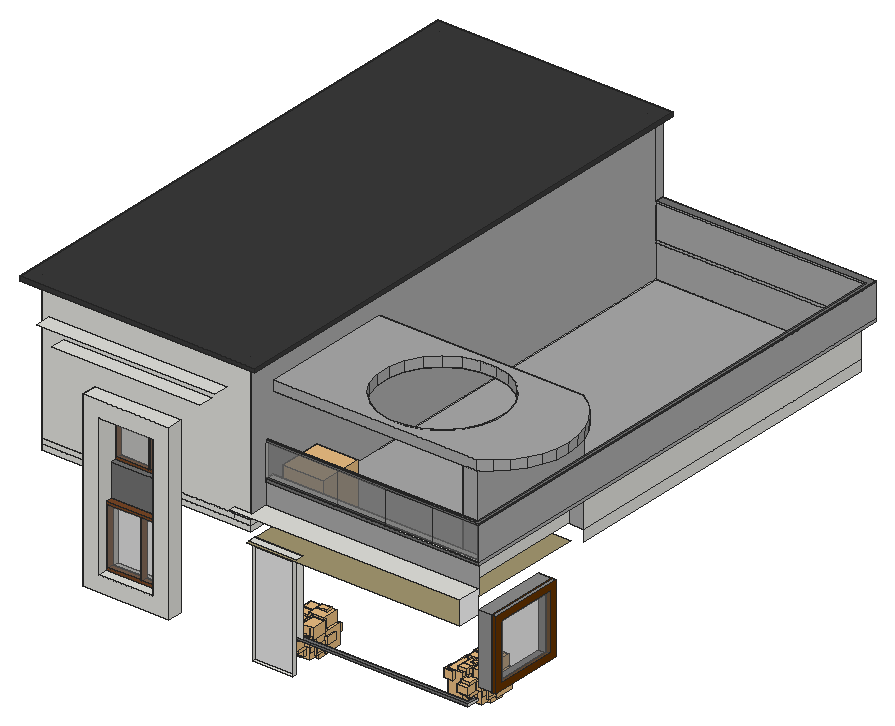
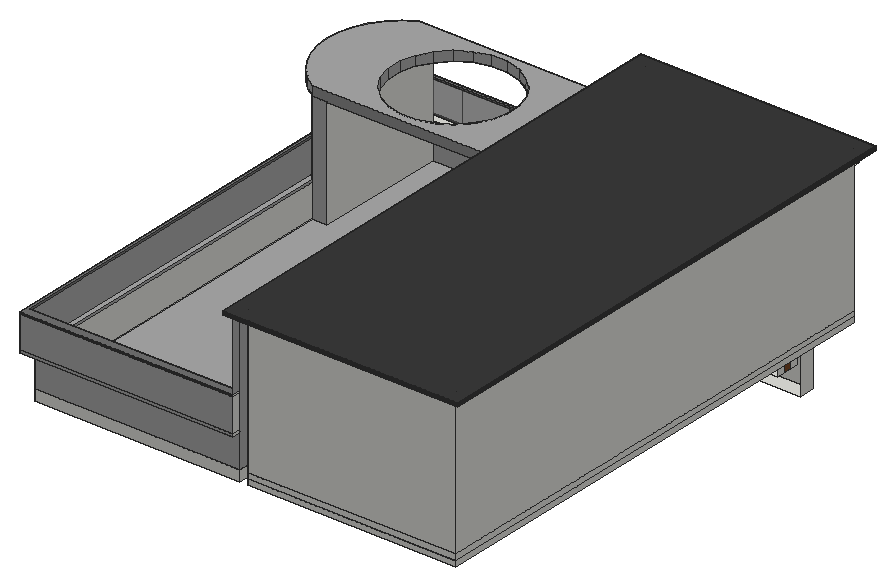
# SketchUp Ruby script. Lengths in inches.
U = 1.inch
M = Sketchup.active_model
def pt(a) = Geom::Point3d.new(a.map { |v| v * U })
def face(e, loops, mat)
  f = e.add_face(loops[0].map { |a| pt(a) })
  loops[1..].each { |l| e.add_face(l.map { |a| pt(a) }).erase! }
  f.material = f.back_material = mat if mat
  f
end
# faces: each face lists its corners as indices into pts; further lists are holes
def faces(e, pts, list, mat = nil) = list.each { |f| face(e, (f[0].is_a?(Array) ? f : [f]).map { |l| l.map { |i| pts[i] } }, mat) }
# xy, xz, yz: faces in a plane at the given z, y or x. An outline is a flat list of corners, or four numbers for a rectangle; further outlines are holes
def ring(l) = l.size == 4 ? [[l[0], l[1]], [l[2], l[1]], [l[2], l[3]], [l[0], l[3]]] : l.each_slice(2).to_a
def flat(e, list, mat, &to3) = list.each { |f| face(e, (f[0].is_a?(Array) ? f : [f]).map { |l| ring(l).map { |u, v| to3.(u, v) } }, mat) }
def xy(e, z, list, mat = nil) = flat(e, list, mat) { |x, y| [x, y, z] }
def xz(e, y, list, mat = nil) = flat(e, list, mat) { |x, z| [x, y, z] }
def yz(e, x, list, mat = nil) = flat(e, list, mat) { |y, z| [x, y, z] }
def lines(e, pts, list) = list.each { |a, b| e.add_line(pt(pts[a]), pt(pts[b])) }
# prism: a flat outline (further loops are holes) pulled along v
def prism(e, loops, v, mat = nil)
  f = face(e, loops, mat); d = Geom::Vector3d.new(v.map { |x| x * U })
  f.pushpull(f.normal.samedirection?(d) ? d.length : -d.length)
end
def box(e, o, s, mat = nil) = prism(e, [[o, [o[0] + s[0], o[1], o[2]], [o[0] + s[0], o[1] + s[1], o[2]], [o[0], o[1] + s[1], o[2]]]], [0, 0, s[2]], mat)
def at(x, y, z, deg = 0) = Geom::Transformation.translation(pt([x, y, z])) * Geom::Transformation.rotation(ORIGIN, Z_AXIS, deg.degrees)
def axes(o, x, y, z) = Geom::Transformation.new([*x, 0, *y, 0, *z, 0, *pt(o).to_a, 1])
def part(name) = M.definitions.add(name)
# library, detail: a bought-in or finely detailed component or shape, given as its bounding box
def library(name, o, s) = part(name).tap { |d| box(d.entities, o, s) }
def detail(e, o, s) = box(e.add_group.entities, o, s)
def put(e, d, t, mat = nil) = e.add_instance(d, t).tap { |i| i.material = mat if mat }
def group(e, t, mat = nil) = e.add_group.tap { |g| g.transformation = t; g.material = mat if mat }.entities
root = M.entities
M.materials.add("Bud_1").color = [142, 54, 77]
M.materials.add("Bud_2").color = [160, 82, 113]
M.materials.add("Bud_3").color = [186, 134, 155]
M.materials.add("Peony_Br1").color = [26, 30, 15]
M.materials.add("[Color C08]1").color = [102, 51, 0]
M.materials.add("[Color M00]").color = [255, 255, 255]
M.materials.add("[Color M03]").color = [170, 170, 170]
M.materials.add("[Color M04]").color = [142, 142, 142]
M.materials.add("[Color M05]").color = [114, 114, 114]
M.materials.add("[Color M07]").color = [58, 58, 58]
M.materials.add("[Sketchy Scales]").color = [229, 229, 229]
M.materials.add("[Translucent Glass Gray]").color = [128, 128, 128]
M.materials["[Translucent Glass Gray]"].alpha = 0.5
M.materials.add("[Wood Lumber ButtJoined]").color = [164, 152, 112]
M.materials.add("[Wood Veneer 01]").color = [120, 70, 37]
c1 = library("Group\#61",[-54.58,-83.54,30.99],[209.74,138.81,269.85])
c2 = library("Group\#54",[-161.17,-232.45,32.75],[152.53,236.06,399.97])
c3 = library("Group\#58",[-62.72,-147.62,57.55],[93.45,86.61,60.22])
c4 = library("Group\#55",[6.78,-176.96,61.53],[128.84,205.63,400.02])
c5 = library("Group\#60",[-32.97,-25.89,74.09],[206.79,187.79,274.23])
c6 = library("Group\#56",[-1.6875,-94.42,75.86],[134.92,113.41,305.11])
c7 = library("Group\#57",[-60.84,-159.99,77.97],[92.87,130.98,190.36])
c8 = library("Group\#59",[-84.97,-34.6875,78.05],[116.39,151.55,263.18])
c9 = library("Group\#14",[-14.51,-199.73,94.2],[105.22,97.74,77.03])
c10 = library("Group\#13",[-28.1,-125.85,106.48],[194.72,128.52,261.01])
c11 = library("Group\#15",[-24.89,-182.93,111.64],[113.72,173.94,173.74])
c12 = library("Group\#51",[-39.88,-92.9,113.08],[80.99,54.06,154.09])
c13 = library("Group\#36",[-37.32,-33.18,117.69],[148.47,104.95,286.6])
c14 = library("Group\#6",[-53.74,7.67,120.98],[106.95,236.74,251.98])
c15 = library("Group\#32",[-118.71,-26.72,138.49],[113,166.64,338.37])
c16 = library("Group\#30",[-110.02,-64.26,144.44],[128.07,118.55,275.77])
c17 = library("Group\#18",[-21.74,-164.88,146.75],[158.66,158.69,243.45])
c18 = library("Group\#9",[-100.48,19.53,147.87],[113.05,111.28,101.19])
c19 = library("Group\#12",[70.77,-125.64,148.84],[102.7,108.07,96.82])
c20 = library("Group\#34",[-136.13,-14.65,175.64],[147.69,202.17,192.49])
c21 = library("Group\#17",[2.57,-271.06,187.04],[93.4,209.89,191.26])
c22 = library("Group\#125",[134.07,-35.59,197.42],[66.93,108.39,101.45])
c23 = library("Group\#42",[-81.93,-128.91,211.16],[107.53,90.8,94.63])
c24 = library("Group\#28",[-168.05,-105.3,214.4],[173.05,109.74,165.51])
c25 = library("Group\#24",[-86.85,-171.15,214.86],[148.39,157.28,240.38])
c26 = library("Group\#124",[44.02,93.6,218.34],[115.22,101.76,105.18])
c27 = library("Group\#38",[-20.13,5.57,225.44],[155.68,162.88,267.12])
c28 = library("Group\#16",[-7.79,-309.02,238.22],[108.5,93.72,102.44])
c29 = library("Group\#126",[-107.16,-137.18,245.54],[76.51,112.05,84.97])
c30 = library("Group\#19",[51.13,-202.98,245.86],[103.83,96.91,120.11])
c31 = library("Group\#48",[1.16,-23.73,246.66],[101.27,126.17,86.62])
c32 = library("Group\#10",[-54.85,-171.1875,247.55],[90.72,132.3,71.07])
c33 = library("Group\#50",[-94.36,-157.31,255.2],[101.84,115.08,71.07])
c34 = library("Group\#31",[-124.14,3.49,256.66],[120.45,70.64,46.18])
c35 = library("Group\#33",[-159.97,129.63,257.39],[89.36,80.73,106.4])
c36 = library("Group\#39",[-80.73,-182.31,261.98],[90.74,132.73,71.97])
c37 = library("Group\#53",[-39.96,0.65,262.91],[71.32,151.8,74.06])
c38 = library("Group\#22",[-80.82,10.33,268.03],[91.87,74,84.35])
c39 = library("Group\#45",[-10.36,3.03,272.26],[79.07,139.88,53.94])
c40 = library("Group\#44",[-45.26,-82.43,273.6875],[73.19,105.45,181.93])
c41 = library("Group\#47",[-40.71,1.11,275.78],[91.4,147.63,75.64])
c42 = library("Group\#27",[-210.125,-102.4375,276.88],[51.54,90.91,87.28])
c43 = library("Group\#123",[-19.56,232.65,283.18],[66.82,42.19,66.65])
c44 = library("Group\#41",[-39.42,-209.09,286.91],[66.94,168.34,116.98])
c45 = library("Group\#8",[-56.625,3.66,294.95],[88.3,152.82,59.14])
c46 = library("Group\#49",[-53.8125,-212.33,295.34],[68.49,139.76,73.67])
c47 = library("Group\#46",[24.16,-5.45,296.62],[84.08,128.04,53.21])
c48 = library("Group\#25",[-191.98,-250.23,297.57],[97.9,89.36,114.5])
c49 = library("Group\#52",[-59.78,14.09,300.39],[101.06,171.37,85.05])
c50 = library("Group\#20",[111.16,-90.29,303.89],[49.95,90,76.18])
c51 = library("Group\#26",[-192.01,-26.24,304.89],[187.25,107.21,53.21])
c52 = library("Group\#40",[-75.53,-189.01,309.71],[68.94,147.24,88.69])
c53 = library("Group\#43",[-21.54,14.12,313.18],[84.79,137.02,109.55])
c54 = library("Group\#11",[-161.51,-101.97,314.73],[172.81,108.71,69.27])
c55 = library("Group\#7",[-49.75,139.84,314.95],[22.11,22.61,22.06])
c56 = library("Group\#21",[47.44,-177.11,343.1],[125.1,149.08,142.01])
c57 = library("Group\#29",[-147.09,-43.87,347.03],[63.89,87.81,80.15])
c58 = library("Group\#35",[-5.59,-15.12,374.79],[85.57,86.81,59.51])
c59 = library("Group\#127",[-126.0625,56.51,376.27],[112.05,106.35,108.99])
c60 = library("Group\#23",[-75.58,-212.0625,396.64],[87.14,69.73,75.82])
c61 = library("Group\#37",[-6.61,93.85,461.94],[98.68,62.42,49.38])
c62 = part("Group\#3")
xy(c62.entities,0,[[0,0,47.875,6]])
xy(c62.entities,1.8,[[1.8,0,30.57,6],[31.73,0,46.07,6]],"[Wood Veneer 01]")
xy(c62.entities,34.82,[[1.8,0,30.57,6],[31.73,0,46.07,6]])
xy(c62.entities,36.625,[[0,0,47.875,6]],"[Wood Veneer 01]")
xz(c62.entities,0,[[1.8,1.8,30.57,34.82],[31.73,1.8,46.07,34.82]],"[Translucent Glass Gray]")
xz(c62.entities,0,[[[0,0,47.875,36.625],[1.8,1.8,30.57,34.82],[31.73,1.8,46.07,34.82]]],"[Wood Veneer 01]")
xz(c62.entities,6,[[[0,0,47.875,36.625],[1.8,1.8,30.57,34.82],[31.73,1.8,46.07,34.82]]],"[Wood Veneer 01]")
yz(c62.entities,0,[[0,0,6,36.625]],"[Wood Veneer 01]")
yz(c62.entities,1.8,[[0,1.8,6,34.82]],"[Wood Veneer 01]")
yz(c62.entities,30.57,[[0,1.8,6,34.82]],"[Wood Veneer 01]")
yz(c62.entities,31.73,[[0,1.8,6,34.82]],"[Wood Veneer 01]")
yz(c62.entities,46.07,[[0,1.8,6,34.82]],"[Wood Veneer 01]")
yz(c62.entities,47.875,[[0,0,6,36.625]],"[Wood Veneer 01]")
c63 = library("Group3\#1",[-239.85,50.56,0],[44.98,46.36,46.21])
xy(root,196.02,[[254.52,161.01,299.22,164.69]])
xy(root,212.85,[[78.82,148.57,172.73,165.13]])
xy(root,223.41,[[465.0625,207.39,484.125,290.14]],"[Color M04]")
xy(root,228,[[250.5,169.32,250.5,173.51,480.43,173.51,480.43,182.19,484.125,182.19,484.125,169.32]])
xy(root,230.3125,[[250.5,169.32,484.125,169.32,484.125,182.19,480.43,182.19,480.43,173.51,250.5,173.51]],"[Color M05]")
xy(root,230.45,[[96.42,148.57,155.13,174.8125]])
xy(root,291.4375,[[351.29,333.375,432.1,339.375]])
xy(root,292.62,[[96.42,165.13,155.13,174.8125]],"[Color M05]")
xy(root,299.35,[[465.0625,207.39,484.125,290.14]],"[Color M04]")
xy(root,308.23,[[254.52,161.01,299.22,164.69]])
xy(root,312,[[250.5,157.82,250.5,333.375,465.0625,333.375,465.0625,182.19,484.125,182.19,484.125,157.82]],"[Wood Lumber ButtJoined]")
xy(root,312.25,[[250.5,161.01,303.24,169.32]])
xy(root,318,[[13.125,174.8125,241.5,718.875]])
xy(root,324,[[13.125,174.8125,241.5,718.875]])
xy(root,324,[[250.5,194.375,458.16,194.375,458.16,339.375,475.125,339.375,475.125,718.875,250.5,718.875]],"[Color M03]")
xy(root,334.28,[[96.42,165.13,155.13,174.8125]],"[Color M05]")
xy(root,337.3125,[[232.4375,157.82,484.125,157.82,484.125,184.0625,250.5,184.0625,250.5,165.13,232.4375,165.13]])
xy(root,360,[[250.5,184.0625,250.5,194.375,475.125,194.375,475.125,718.875,250.5,718.875,250.5,727.875,484.125,727.875,484.125,184.0625]])
xy(root,363,[[250.5,184.0625,250.5,186.625,480.6875,186.625,480.6875,718.875,250.5,718.875,250.5,727.875,484.125,727.875,484.125,184.0625],[250.5,186.625,480.6875,194.375]])
xy(root,363,[[475.125,194.375,480.6875,718.875]],"[Color M03]")
xy(root,384.1,[[96.42,148.57,155.13,174.8125]])
xy(root,399,[[250.5,184.0625,250.5,186.625,480.6875,186.625,480.6875,718.875,250.5,718.875,250.5,727.875,484.125,727.875,484.125,184.0625]])
xy(root,401,[[250.5,184.0625,484.125,184.0625,484.125,727.875,250.5,727.875,250.5,718.875,480.6875,718.875,480.6875,186.625,250.5,186.625]],"[Color M05]")
xy(root,401.7,[[78.82,148.57,172.73,165.13]])
xy(root,435.66,[[44.86,148.38,206.69,165.13]])
xy(root,445.0625,[[[250.5,194.375,458.16,339.375],[371.27,202.37,388.16,202.8,404.375,207.59,418.79,216.42,430.43,228.67,438.51,243.52,442.46,259.95,442.03,276.85,437.24,293.0625,428.42,307.48,416.16,319.12,401.3125,327.2,384.88,331.15,367.98,330.72,351.77,325.93,337.35,317.1,325.71,304.85,317.64,290,313.68,273.57,314.11,256.67,318.9,240.46,327.73,226.04,339.98,214.4,354.83,206.32]],[458.16,194.375,473.7,194.375,475.125,195.34,475.125,338.41,473.7,339.375,458.16,339.375],[473.7,194.375,475.125,194.375,475.125,195.34],[475.125,195.34,475.125,338.41,485.88,331.15,496.42,320.91,504.98,308.96,511.3,295.69,515.17,281.51,516.47,266.875,515.17,252.24,511.3,238.06,504.98,224.79,496.42,212.84,485.88,202.6],[475.125,338.41,475.125,339.375,473.7,339.375]])
xy(root,452.06,[[28.46,148.38,223.09,165.13]])
xy(root,455.625,[[[250.5,194.375,473.7,194.375,485.88,202.6,496.42,212.84,504.98,224.79,511.3,238.06,515.17,252.24,516.47,266.875,515.17,281.51,511.3,295.69,504.98,308.96,496.42,320.91,485.88,331.15,473.7,339.375,250.5,339.375],[371.27,202.37,354.83,206.32,339.98,214.4,327.73,226.04,318.9,240.46,314.11,256.67,313.68,273.57,317.64,290,325.71,304.85,337.35,317.1,351.77,325.93,367.98,330.72,384.88,331.15,401.3125,327.2,416.16,319.12,428.42,307.48,437.24,293.0625,442.03,276.85,442.46,259.95,438.51,243.52,430.43,228.67,418.79,216.42,404.375,207.59,388.16,202.8]]],"[Color M03]")
xy(root,480,[[0,160.63,13.125,165.13],[13.125,160.63,241.5,165.13],[241.5,160.63,257.4375,165.13],[0,165.13,4.125,733.3125],[[4.125,165.13,250.5,727.875],[13.125,174.8125,241.5,718.875]],
  [250.5,165.13,257.4375,718.875],[250.5,718.875,257.4375,733.3125],[4.125,727.875,250.5,733.3125]])
xy(root,484,[[0,160.63,257.4375,733.3125]],"[Color M07]")
xz(root,148.57,[[[78.82,212.85,172.73,401.7],[96.42,230.45,155.13,384.1]]])
xz(root,160.63,[[0,480,257.4375,484]],"[Color M07]")
xz(root,164.69,[[254.52,196.02,299.22,308.23]],"[Sketchy Scales]")
xz(root,165.13,[[96.42,292.62,155.13,334.28]],"[Color M05]")
xz(root,169.32,[[250.5,230.3125,303.24,312.25]])
xz(root,169.32,[[250.5,228,303.24,230.3125],[303.24,228,484.125,230.3125]],"[Color M05]")
xz(root,173.51,[[250.5,228,480.43,230.3125]])
xz(root,174.8125,[[13.125,312,241.5,318],[13.125,318,223.3125,324],[223.3125,318,241.5,324],[[13.125,324,241.5,480],[96.42,334.28,155.13,384.1]]])
xz(root,182.19,[[480.43,228,484.125,230.3125]])
xz(root,184.0625,[[250.5,337.3125,484.125,360]],"[Color M03]")
xz(root,184.0625,[[250.5,360,484.125,363],[250.5,399,484.125,401]],"[Color M05]")
xz(root,184.0625,[[250.5,363,330.1875,399],[330.1875,363,382.81,399],[382.81,363,433.47,399],[433.47,363,484.125,399]],"[Translucent Glass Gray]")
xz(root,186.625,[[250.5,399,480.6875,401]],"[Color M05]")
xz(root,186.625,[[250.5,363,480.6875,399]],"[Translucent Glass Gray]")
xz(root,194.375,[[250.5,360,458.16,363],[458.16,360,475.125,363]])
xz(root,194.375,[[250.5,324,458.16,360],[458.16,363,475.125,445.0625],[250.5,445.0625,473.7,455.625]],"[Color M03]")
xz(root,207.39,[[465.0625,223.41,484.125,299.35]],"[Color M04]")
xz(root,290.14,[[465.0625,223.41,484.125,299.35]],"[Color M04]")
xz(root,339.375,[[458.16,324,475.125,445.0625]],"[Color M03]")
xz(root,339.375,[[250.5,445.0625,473.7,455.625]],"[Color M04]")
xz(root,718.875,[[13.125,312,241.5,318],[250.5,312,475.125,324],[13.125,318,241.5,324],[13.125,324,241.5,480]])
xz(root,718.875,[[250.5,324,475.125,360],[250.5,360,475.125,363],[250.5,363,480.6875,399],[250.5,399,480.6875,401]],"[Color M03]")
xz(root,727.875,[[250.5,360,484.125,363],[250.5,363,484.125,399]],"[Color M03]")
xz(root,727.875,[[250.5,399,484.125,401]],"[Color M07]")
xz(root,733.3125,[[0,480,257.4375,484]],"[Color M07]")
yz(root,0,[[160.63,480,733.3125,484]],"[Color M07]")
yz(root,13.125,[[174.8125,312,718.875,318],[174.8125,318,718.875,324],[174.8125,324,718.875,480]])
yz(root,78.82,[[148.57,212.85,165.13,401.7]])
yz(root,96.42,[[148.57,230.45,174.8125,230.45,174.8125,292.62,165.13,292.62,165.13,334.28,174.8125,334.28,174.8125,384.1,148.57,384.1]])
yz(root,155.13,[[148.57,230.45,148.57,384.1,174.8125,384.1,174.8125,334.28,165.13,334.28,165.13,292.62,174.8125,292.62,174.8125,230.45]])
yz(root,172.73,[[148.57,212.85,165.13,401.7]])
yz(root,241.5,[[174.8125,312,718.875,318],[174.8125,318,718.875,324],[174.8125,324,718.875,480]])
yz(root,250.5,[[169.32,228,173.51,230.3125],[161.01,312,169.32,312.25],[339.375,312,718.875,324],[184.0625,360,194.375,363],[718.875,360,727.875,363],
  [184.0625,363,186.625,399],[718.875,363,727.875,399],[184.0625,399,186.625,401],[718.875,399,727.875,401]])
yz(root,250.5,[[[194.375,324,718.875,324,718.875,480,165.13,480,165.13,337.3125,184.0625,337.3125,184.0625,401,186.625,401,186.625,363,194.375,363],[194.375,445.0625,339.375,455.625]],[718.875,401,727.875,480]],"[Color M03]")
yz(root,254.52,[[161.01,196.02,164.69,308.23]])
yz(root,257.4375,[[160.63,480,733.3125,484]],"[Color M07]")
yz(root,299.22,[[161.01,196.02,164.69,308.23]])
yz(root,458.16,[[194.375,324,339.375,445.0625]])
yz(root,475.125,[[339.375,312,718.875,324],[339.375,324,718.875,360],[194.375,360,339.375,363]])
yz(root,475.125,[[339.375,360,718.875,363],[194.375,363,339.375,445.0625]],"[Color M03]")
yz(root,480.43,[[173.51,228,182.19,230.3125]])
yz(root,480.6875,[[186.625,363,718.875,399]],"[Color M03]")
yz(root,480.6875,[[186.625,399,718.875,401]],"[Color M05]")
yz(root,484.125,[[169.32,228,182.19,230.3125]])
yz(root,484.125,[[157.82,312,182.19,312,182.19,324,184.0625,337.3125,157.82,337.3125]],"[Color M00]")
yz(root,484.125,[[184.0625,360,727.875,363],[184.0625,363,727.875,399]],"[Color M03]")
yz(root,484.125,[[184.0625,399,727.875,401]],"[Color M07]")
p = [[485.88,202.6,455.625],[473.7,194.375,455.625],[473.7,194.375,445.0625],[475.125,195.34,445.0625],[485.88,202.6,445.0625],[354.83,206.32,455.625],
  [371.27,202.37,455.625],[371.27,202.37,445.0625],[354.83,206.32,445.0625],[388.16,202.8,455.625],[388.16,202.8,445.0625],[496.42,212.84,455.625],
  [496.42,212.84,445.0625],[404.375,207.59,455.625],[404.375,207.59,445.0625],[339.98,214.4,455.625],[339.98,214.4,445.0625],[418.79,216.42,455.625],
  [418.79,216.42,445.0625],[504.98,224.79,455.625],[504.98,224.79,445.0625],[327.73,226.04,455.625],[327.73,226.04,445.0625],[430.43,228.67,455.625],
  [430.43,228.67,445.0625],[511.3,238.06,455.625],[511.3,238.06,445.0625],[318.9,240.46,455.625],[318.9,240.46,445.0625],[438.51,243.52,455.625],
  [438.51,243.52,445.0625],[515.17,252.24,455.625],[515.17,252.24,445.0625],[314.11,256.67,455.625],[314.11,256.67,445.0625],[442.46,259.95,455.625],
  [442.46,259.95,445.0625],[516.47,266.875,455.625],[516.47,266.875,445.0625],[313.68,273.57,455.625],[313.68,273.57,445.0625],[442.03,276.85,455.625],
  [442.03,276.85,445.0625],[515.17,281.51,455.625],[515.17,281.51,445.0625],[317.64,290,455.625],[317.64,290,445.0625],[437.24,293.0625,455.625],
  [437.24,293.0625,445.0625],[511.3,295.69,455.625],[511.3,295.69,445.0625],[325.71,304.85,455.625],[325.71,304.85,445.0625],[428.42,307.48,455.625],
  [428.42,307.48,445.0625],[504.98,308.96,455.625],[504.98,308.96,445.0625],[337.35,317.1,455.625],[337.35,317.1,445.0625],[416.16,319.12,455.625],
  [416.16,319.12,445.0625],[496.42,320.91,455.625],[496.42,320.91,445.0625],[351.77,325.93,455.625],[351.77,325.93,445.0625],[401.3125,327.2,455.625],
  [401.3125,327.2,445.0625],[485.88,331.15,455.625],[485.88,331.15,445.0625],[367.98,330.72,455.625],[367.98,330.72,445.0625],[384.88,331.15,455.625],
  [384.88,331.15,445.0625],[473.7,339.375,455.625],[475.125,338.41,445.0625],[473.7,339.375,445.0625],[241.5,174.8125,480],[241.5,174.8125,484],
  [241.5,718.875,480],[241.5,718.875,484],[13.125,174.8125,480],[13.125,174.8125,484],[13.125,718.875,480],[13.125,718.875,484]]
faces(root,p,[[0,1,2,3,4],[5,6,7,8],[6,9,10,7],[11,0,4,12],[9,13,14,10],[15,5,8,16],[13,17,18,14],[19,11,12,20],
  [21,15,16,22],[17,23,24,18],[25,19,20,26],[27,21,22,28],[23,29,30,24],[31,25,26,32],[33,27,28,34],[29,35,36,30],
  [37,31,32,38],[39,33,34,40],[35,41,42,36],[43,37,38,44],[45,39,40,46],[41,47,48,42],[49,43,44,50],[51,45,46,52],
  [47,53,54,48],[55,49,50,56],[57,51,52,58],[53,59,60,54],[61,55,56,62],[63,57,58,64],[59,65,66,60],[67,61,62,68],
  [69,63,64,70],[65,71,72,66],[71,69,70,72],[73,67,68,74,75]],"[Color M03]")
lines(root,p,[[76,77],[78,79],[80,81],[82,83]])
put(root,c1,axes([279.06,209.92,192.1875],[0.1075,0,0],[0,0.1075,0],[0,0,0.0774]),"Peony_Br1")
put(root,c1,axes([441.92,241.33,192.1875],[0.1075,0,0],[0,0.1075,0],[0,0,0.0774]),"Peony_Br1")
put(root,c2,axes([279.06,209.92,192.1875],[0.1075,0,0],[0,0.1075,0],[0,0,0.0774]),"Peony_Br1")
put(root,c2,axes([441.92,241.33,192.1875],[0.1075,0,0],[0,0.1075,0],[0,0,0.0774]),"Peony_Br1")
put(root,c3,axes([279.06,209.92,192.1875],[0.1075,0,0],[0,0.1075,0],[0,0,0.0774]),"Bud_2")
put(root,c3,axes([441.92,241.33,192.1875],[0.1075,0,0],[0,0.1075,0],[0,0,0.0774]),"Bud_2")
put(root,c4,axes([279.06,209.92,192.1875],[0.1075,0,0],[0,0.1075,0],[0,0,0.0774]),"Peony_Br1")
put(root,c4,axes([441.92,241.33,192.1875],[0.1075,0,0],[0,0.1075,0],[0,0,0.0774]),"Peony_Br1")
put(root,c5,axes([279.06,209.92,192.1875],[0.1075,0,0],[0,0.1075,0],[0,0,0.0774]),"Peony_Br1")
put(root,c5,axes([441.92,241.33,192.1875],[0.1075,0,0],[0,0.1075,0],[0,0,0.0774]),"Peony_Br1")
put(root,c6,axes([279.06,209.92,192.1875],[0.1075,0,0],[0,0.1075,0],[0,0,0.0774]),"Peony_Br1")
put(root,c6,axes([441.92,241.33,192.1875],[0.1075,0,0],[0,0.1075,0],[0,0,0.0774]),"Peony_Br1")
put(root,c7,axes([279.06,209.92,192.1875],[0.1075,0,0],[0,0.1075,0],[0,0,0.0774]),"Peony_Br1")
put(root,c7,axes([441.92,241.33,192.1875],[0.1075,0,0],[0,0.1075,0],[0,0,0.0774]),"Peony_Br1")
put(root,c8,axes([279.06,209.92,192.1875],[0.1075,0,0],[0,0.1075,0],[0,0,0.0774]),"Peony_Br1")
put(root,c8,axes([441.92,241.33,192.1875],[0.1075,0,0],[0,0.1075,0],[0,0,0.0774]),"Peony_Br1")
put(root,c9,axes([279.06,209.92,192.1875],[0.1075,0,0],[0,0.1075,0],[0,0,0.0774]),"Bud_2")
put(root,c9,axes([441.92,241.33,192.1875],[0.1075,0,0],[0,0.1075,0],[0,0,0.0774]),"Bud_2")
put(root,c10,axes([279.06,209.92,192.1875],[0.1075,0,0],[0,0.1075,0],[0,0,0.0774]),"Peony_Br1")
put(root,c10,axes([441.92,241.33,192.1875],[0.1075,0,0],[0,0.1075,0],[0,0,0.0774]),"Peony_Br1")
put(root,c11,axes([279.06,209.92,192.1875],[0.1075,0,0],[0,0.1075,0],[0,0,0.0774]),"Peony_Br1")
put(root,c11,axes([441.92,241.33,192.1875],[0.1075,0,0],[0,0.1075,0],[0,0,0.0774]),"Peony_Br1")
put(root,c12,axes([279.06,209.92,192.1875],[0.1075,0,0],[0,0.1075,0],[0,0,0.0774]),"Peony_Br1")
put(root,c12,axes([441.92,241.33,192.1875],[0.1075,0,0],[0,0.1075,0],[0,0,0.0774]),"Peony_Br1")
put(root,c13,axes([279.06,209.92,192.1875],[0.1075,0,0],[0,0.1075,0],[0,0,0.0774]),"Peony_Br1")
put(root,c13,axes([441.92,241.33,192.1875],[0.1075,0,0],[0,0.1075,0],[0,0,0.0774]),"Peony_Br1")
put(root,c14,axes([279.06,209.92,192.1875],[0.1075,0,0],[0,0.1075,0],[0,0,0.0774]),"Peony_Br1")
put(root,c14,axes([441.92,241.33,192.1875],[0.1075,0,0],[0,0.1075,0],[0,0,0.0774]),"Peony_Br1")
put(root,c15,axes([279.06,209.92,192.1875],[0.1075,0,0],[0,0.1075,0],[0,0,0.0774]),"Peony_Br1")
put(root,c15,axes([441.92,241.33,192.1875],[0.1075,0,0],[0,0.1075,0],[0,0,0.0774]),"Peony_Br1")
put(root,c16,axes([279.06,209.92,192.1875],[0.1075,0,0],[0,0.1075,0],[0,0,0.0774]),"Peony_Br1")
put(root,c16,axes([441.92,241.33,192.1875],[0.1075,0,0],[0,0.1075,0],[0,0,0.0774]),"Peony_Br1")
put(root,c17,axes([279.06,209.92,192.1875],[0.1075,0,0],[0,0.1075,0],[0,0,0.0774]),"Peony_Br1")
put(root,c17,axes([441.92,241.33,192.1875],[0.1075,0,0],[0,0.1075,0],[0,0,0.0774]),"Peony_Br1")
put(root,c18,axes([279.06,209.92,192.1875],[0.1075,0,0],[0,0.1075,0],[0,0,0.0774]),"Bud_1")
put(root,c18,axes([441.92,241.33,192.1875],[0.1075,0,0],[0,0.1075,0],[0,0,0.0774]),"Bud_1")
put(root,c19,axes([279.06,209.92,192.1875],[0.1075,0,0],[0,0.1075,0],[0,0,0.0774]),"Bud_2")
put(root,c19,axes([441.92,241.33,192.1875],[0.1075,0,0],[0,0.1075,0],[0,0,0.0774]),"Bud_2")
put(root,c20,axes([279.06,209.92,192.1875],[0.1075,0,0],[0,0.1075,0],[0,0,0.0774]),"Peony_Br1")
put(root,c20,axes([441.92,241.33,192.1875],[0.1075,0,0],[0,0.1075,0],[0,0,0.0774]),"Peony_Br1")
put(root,c21,axes([279.06,209.92,192.1875],[0.1075,0,0],[0,0.1075,0],[0,0,0.0774]),"Peony_Br1")
put(root,c21,axes([441.92,241.33,192.1875],[0.1075,0,0],[0,0.1075,0],[0,0,0.0774]),"Peony_Br1")
put(root,c22,axes([279.06,209.92,192.1875],[0.1075,0,0],[0,0.1075,0],[0,0,0.0774]),"Bud_2")
put(root,c22,axes([441.92,241.33,192.1875],[0.1075,0,0],[0,0.1075,0],[0,0,0.0774]),"Bud_2")
put(root,c23,axes([279.06,209.92,192.1875],[0.1075,0,0],[0,0.1075,0],[0,0,0.0774]),"Peony_Br1")
put(root,c23,axes([441.92,241.33,192.1875],[0.1075,0,0],[0,0.1075,0],[0,0,0.0774]),"Peony_Br1")
put(root,c24,axes([279.06,209.92,192.1875],[0.1075,0,0],[0,0.1075,0],[0,0,0.0774]),"Peony_Br1")
put(root,c24,axes([441.92,241.33,192.1875],[0.1075,0,0],[0,0.1075,0],[0,0,0.0774]),"Peony_Br1")
put(root,c25,axes([279.06,209.92,192.1875],[0.1075,0,0],[0,0.1075,0],[0,0,0.0774]),"Peony_Br1")
put(root,c25,axes([441.92,241.33,192.1875],[0.1075,0,0],[0,0.1075,0],[0,0,0.0774]),"Peony_Br1")
put(root,c26,axes([279.06,209.92,192.1875],[0.1075,0,0],[0,0.1075,0],[0,0,0.0774]),"Bud_2")
put(root,c26,axes([441.92,241.33,192.1875],[0.1075,0,0],[0,0.1075,0],[0,0,0.0774]),"Bud_2")
put(root,c27,axes([279.06,209.92,192.1875],[0.1075,0,0],[0,0.1075,0],[0,0,0.0774]),"Peony_Br1")
put(root,c27,axes([441.92,241.33,192.1875],[0.1075,0,0],[0,0.1075,0],[0,0,0.0774]),"Peony_Br1")
put(root,c28,axes([279.06,209.92,192.1875],[0.1075,0,0],[0,0.1075,0],[0,0,0.0774]),"Bud_2")
put(root,c28,axes([441.92,241.33,192.1875],[0.1075,0,0],[0,0.1075,0],[0,0,0.0774]),"Bud_2")
put(root,c29,axes([279.06,209.92,192.1875],[0.1075,0,0],[0,0.1075,0],[0,0,0.0774]),"Peony_Br1")
put(root,c29,axes([441.92,241.33,192.1875],[0.1075,0,0],[0,0.1075,0],[0,0,0.0774]),"Peony_Br1")
put(root,c30,axes([279.06,209.92,192.1875],[0.1075,0,0],[0,0.1075,0],[0,0,0.0774]),"Bud_2")
put(root,c30,axes([441.92,241.33,192.1875],[0.1075,0,0],[0,0.1075,0],[0,0,0.0774]),"Bud_2")
put(root,c31,axes([279.06,209.92,192.1875],[0.1075,0,0],[0,0.1075,0],[0,0,0.0774]),"Peony_Br1")
put(root,c31,axes([441.92,241.33,192.1875],[0.1075,0,0],[0,0.1075,0],[0,0,0.0774]),"Peony_Br1")
put(root,c32,axes([279.06,209.92,192.1875],[0.1075,0,0],[0,0.1075,0],[0,0,0.0774]),"Peony_Br1")
put(root,c32,axes([441.92,241.33,192.1875],[0.1075,0,0],[0,0.1075,0],[0,0,0.0774]),"Peony_Br1")
put(root,c33,axes([279.06,209.92,192.1875],[0.1075,0,0],[0,0.1075,0],[0,0,0.0774]),"Peony_Br1")
put(root,c33,axes([441.92,241.33,192.1875],[0.1075,0,0],[0,0.1075,0],[0,0,0.0774]),"Peony_Br1")
put(root,c34,axes([279.06,209.92,192.1875],[0.1075,0,0],[0,0.1075,0],[0,0,0.0774]),"Peony_Br1")
put(root,c34,axes([441.92,241.33,192.1875],[0.1075,0,0],[0,0.1075,0],[0,0,0.0774]),"Peony_Br1")
put(root,c35,axes([279.06,209.92,192.1875],[0.1075,0,0],[0,0.1075,0],[0,0,0.0774]),"Bud_3")
put(root,c35,axes([441.92,241.33,192.1875],[0.1075,0,0],[0,0.1075,0],[0,0,0.0774]),"Bud_3")
put(root,c36,axes([279.06,209.92,192.1875],[0.1075,0,0],[0,0.1075,0],[0,0,0.0774]),"Peony_Br1")
put(root,c36,axes([441.92,241.33,192.1875],[0.1075,0,0],[0,0.1075,0],[0,0,0.0774]),"Peony_Br1")
put(root,c37,axes([279.06,209.92,192.1875],[0.1075,0,0],[0,0.1075,0],[0,0,0.0774]),"Peony_Br1")
put(root,c37,axes([441.92,241.33,192.1875],[0.1075,0,0],[0,0.1075,0],[0,0,0.0774]),"Peony_Br1")
put(root,c38,axes([279.06,209.92,192.1875],[0.1075,0,0],[0,0.1075,0],[0,0,0.0774]),"Peony_Br1")
put(root,c38,axes([441.92,241.33,192.1875],[0.1075,0,0],[0,0.1075,0],[0,0,0.0774]),"Peony_Br1")
put(root,c39,axes([279.06,209.92,192.1875],[0.1075,0,0],[0,0.1075,0],[0,0,0.0774]),"Peony_Br1")
put(root,c39,axes([441.92,241.33,192.1875],[0.1075,0,0],[0,0.1075,0],[0,0,0.0774]),"Peony_Br1")
put(root,c40,axes([279.06,209.92,192.1875],[0.1075,0,0],[0,0.1075,0],[0,0,0.0774]),"Peony_Br1")
put(root,c40,axes([441.92,241.33,192.1875],[0.1075,0,0],[0,0.1075,0],[0,0,0.0774]),"Peony_Br1")
put(root,c41,axes([279.06,209.92,192.1875],[0.1075,0,0],[0,0.1075,0],[0,0,0.0774]),"Peony_Br1")
put(root,c41,axes([441.92,241.33,192.1875],[0.1075,0,0],[0,0.1075,0],[0,0,0.0774]),"Peony_Br1")
put(root,c42,axes([279.06,209.92,192.1875],[0.1075,0,0],[0,0.1075,0],[0,0,0.0774]),"Bud_2")
put(root,c42,axes([441.92,241.33,192.1875],[0.1075,0,0],[0,0.1075,0],[0,0,0.0774]),"Bud_2")
put(root,c43,axes([279.06,209.92,192.1875],[0.1075,0,0],[0,0.1075,0],[0,0,0.0774]),"Bud_2")
put(root,c43,axes([441.92,241.33,192.1875],[0.1075,0,0],[0,0.1075,0],[0,0,0.0774]),"Bud_2")
put(root,c44,axes([279.06,209.92,192.1875],[0.1075,0,0],[0,0.1075,0],[0,0,0.0774]),"Peony_Br1")
put(root,c44,axes([441.92,241.33,192.1875],[0.1075,0,0],[0,0.1075,0],[0,0,0.0774]),"Peony_Br1")
put(root,c45,axes([279.06,209.92,192.1875],[0.1075,0,0],[0,0.1075,0],[0,0,0.0774]),"Peony_Br1")
put(root,c45,axes([441.92,241.33,192.1875],[0.1075,0,0],[0,0.1075,0],[0,0,0.0774]),"Peony_Br1")
put(root,c46,axes([279.06,209.92,192.1875],[0.1075,0,0],[0,0.1075,0],[0,0,0.0774]),"Peony_Br1")
put(root,c46,axes([441.92,241.33,192.1875],[0.1075,0,0],[0,0.1075,0],[0,0,0.0774]),"Peony_Br1")
put(root,c47,axes([279.06,209.92,192.1875],[0.1075,0,0],[0,0.1075,0],[0,0,0.0774]),"Peony_Br1")
put(root,c47,axes([441.92,241.33,192.1875],[0.1075,0,0],[0,0.1075,0],[0,0,0.0774]),"Peony_Br1")
put(root,c48,axes([279.06,209.92,192.1875],[0.1075,0,0],[0,0.1075,0],[0,0,0.0774]),"Bud_1")
put(root,c48,axes([441.92,241.33,192.1875],[0.1075,0,0],[0,0.1075,0],[0,0,0.0774]),"Bud_1")
put(root,c49,axes([279.06,209.92,192.1875],[0.1075,0,0],[0,0.1075,0],[0,0,0.0774]),"Peony_Br1")
put(root,c49,axes([441.92,241.33,192.1875],[0.1075,0,0],[0,0.1075,0],[0,0,0.0774]),"Peony_Br1")
put(root,c50,axes([279.06,209.92,192.1875],[0.1075,0,0],[0,0.1075,0],[0,0,0.0774]),"Bud_1")
put(root,c50,axes([441.92,241.33,192.1875],[0.1075,0,0],[0,0.1075,0],[0,0,0.0774]),"Bud_1")
put(root,c51,axes([279.06,209.92,192.1875],[0.1075,0,0],[0,0.1075,0],[0,0,0.0774]),"Peony_Br1")
put(root,c51,axes([441.92,241.33,192.1875],[0.1075,0,0],[0,0.1075,0],[0,0,0.0774]),"Peony_Br1")
put(root,c52,axes([279.06,209.92,192.1875],[0.1075,0,0],[0,0.1075,0],[0,0,0.0774]),"Peony_Br1")
put(root,c52,axes([441.92,241.33,192.1875],[0.1075,0,0],[0,0.1075,0],[0,0,0.0774]),"Peony_Br1")
put(root,c53,axes([279.06,209.92,192.1875],[0.1075,0,0],[0,0.1075,0],[0,0,0.0774]),"Peony_Br1")
put(root,c53,axes([441.92,241.33,192.1875],[0.1075,0,0],[0,0.1075,0],[0,0,0.0774]),"Peony_Br1")
put(root,c54,axes([279.06,209.92,192.1875],[0.1075,0,0],[0,0.1075,0],[0,0,0.0774]),"Peony_Br1")
put(root,c54,axes([441.92,241.33,192.1875],[0.1075,0,0],[0,0.1075,0],[0,0,0.0774]),"Peony_Br1")
put(root,c55,axes([279.06,209.92,192.1875],[0.1075,0,0],[0,0.1075,0],[0,0,0.0774]),"Bud_2")
put(root,c55,axes([441.92,241.33,192.1875],[0.1075,0,0],[0,0.1075,0],[0,0,0.0774]),"Bud_2")
put(root,c56,axes([279.06,209.92,192.1875],[0.1075,0,0],[0,0.1075,0],[0,0,0.0774]),"Bud_3")
put(root,c56,axes([441.92,241.33,192.1875],[0.1075,0,0],[0,0.1075,0],[0,0,0.0774]),"Bud_3")
put(root,c57,axes([279.06,209.92,192.1875],[0.1075,0,0],[0,0.1075,0],[0,0,0.0774]),"Bud_2")
put(root,c57,axes([441.92,241.33,192.1875],[0.1075,0,0],[0,0.1075,0],[0,0,0.0774]),"Bud_2")
put(root,c58,axes([279.06,209.92,192.1875],[0.1075,0,0],[0,0.1075,0],[0,0,0.0774]),"Bud_2")
put(root,c58,axes([441.92,241.33,192.1875],[0.1075,0,0],[0,0.1075,0],[0,0,0.0774]),"Bud_2")
put(root,c59,axes([279.06,209.92,192.1875],[0.1075,0,0],[0,0.1075,0],[0,0,0.0774]),"Bud_1")
put(root,c59,axes([441.92,241.33,192.1875],[0.1075,0,0],[0,0.1075,0],[0,0,0.0774]),"Bud_1")
put(root,c60,axes([279.06,209.92,192.1875],[0.1075,0,0],[0,0.1075,0],[0,0,0.0774]),"Bud_2")
put(root,c60,axes([441.92,241.33,192.1875],[0.1075,0,0],[0,0.1075,0],[0,0,0.0774]),"Bud_2")
g1 = group(root,at(479.625,207.39,223.41))
xy(g1,0,[[0,0,4.5,82.75]],"[Color M03]")
xy(g1,7.38,[[0,8.04,4.5,74.71]],"[Color C08]1")
xy(g1,68.56,[[0,8.04,4.5,74.71]],"[Color C08]1")
xy(g1,75.9375,[[0,0,4.5,82.75]],"[Color C08]1")
xz(g1,0,[[0,0,4.5,75.9375]],"[Color C08]1")
xz(g1,8.04,[[0,7.38,4.5,68.56]],"[Color C08]1")
xz(g1,74.71,[[0,7.38,4.5,68.56]],"[Color C08]1")
xz(g1,82.75,[[0,0,4.5,75.9375]],"[Color C08]1")
yz(g1,0,[[[0,0,82.75,75.9375],[8.04,7.38,74.71,68.56]]],"[Color C08]1")
yz(g1,4.5,[[[0,0,82.75,75.9375],[8.04,7.38,74.71,68.56]]],"[Color C08]1")
yz(g1,4.5,[[8.04,7.38,74.71,68.56]],"[Translucent Glass Gray]")
put(root,c61,axes([279.06,209.92,192.1875],[0.1075,0,0],[0,0.1075,0],[0,0,0.0774]),"Bud_2")
put(root,c61,axes([441.92,241.33,192.1875],[0.1075,0,0],[0,0.1075,0],[0,0,0.0774]),"Bud_2")
put(root,c62,axes([96.41,158.42,230.45],[1.22653,0,0],[0,1.05966,0],[0,0,1.8705]))
put(root,c63,at(494.22,152.39,324))
put(root,c62,axes([96.41,170.61,334.28],[1.22653,0,0],[0,0.9135,0],[0,0,1.36034]))
